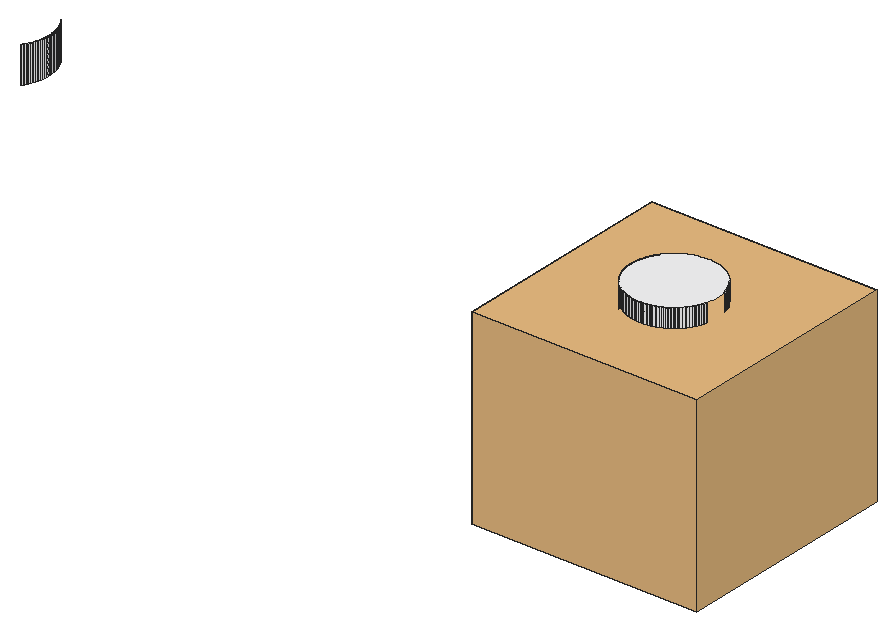
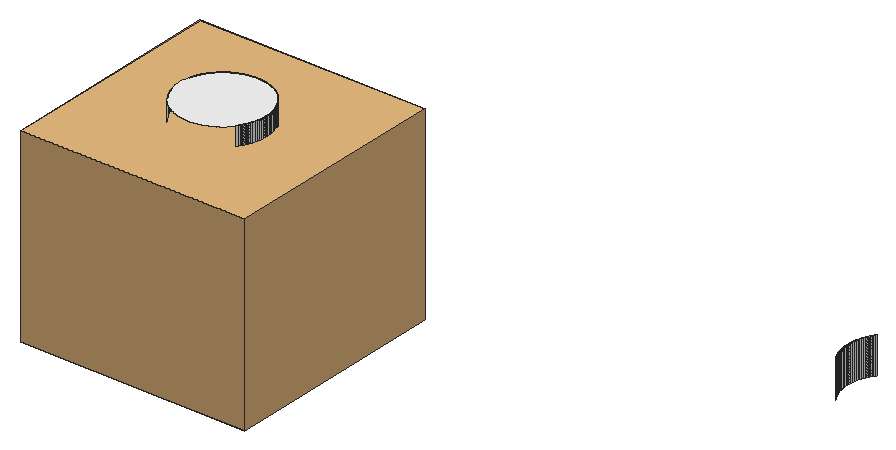
# SketchUp Ruby script. Lengths in inches.
U = 1.inch
M = Sketchup.active_model
def pt(a) = Geom::Point3d.new(a.map { |v| v * U })
def face(e, loops, mat)
  f = e.add_face(loops[0].map { |a| pt(a) })
  loops[1..].each { |l| e.add_face(l.map { |a| pt(a) }).erase! }
  f.material = f.back_material = mat if mat
  f
end
# faces: each face lists its corners as indices into pts; further lists are holes
def faces(e, pts, list, mat = nil) = list.each { |f| face(e, (f[0].is_a?(Array) ? f : [f]).map { |l| l.map { |i| pts[i] } }, mat) }
# xy, xz, yz: faces in a plane at the given z, y or x. An outline is a flat list of corners, or four numbers for a rectangle; further outlines are holes
def ring(l) = l.size == 4 ? [[l[0], l[1]], [l[2], l[1]], [l[2], l[3]], [l[0], l[3]]] : l.each_slice(2).to_a
def flat(e, list, mat, &to3) = list.each { |f| face(e, (f[0].is_a?(Array) ? f : [f]).map { |l| ring(l).map { |u, v| to3.(u, v) } }, mat) }
def xy(e, z, list, mat = nil) = flat(e, list, mat) { |x, y| [x, y, z] }
def xz(e, y, list, mat = nil) = flat(e, list, mat) { |x, z| [x, y, z] }
def yz(e, x, list, mat = nil) = flat(e, list, mat) { |y, z| [x, y, z] }
def lines(e, pts, list) = list.each { |a, b| e.add_line(pt(pts[a]), pt(pts[b])) }
# prism: a flat outline (further loops are holes) pulled along v
def prism(e, loops, v, mat = nil)
  f = face(e, loops, mat); d = Geom::Vector3d.new(v.map { |x| x * U })
  f.pushpull(f.normal.samedirection?(d) ? d.length : -d.length)
end
def box(e, o, s, mat = nil) = prism(e, [[o, [o[0] + s[0], o[1], o[2]], [o[0] + s[0], o[1] + s[1], o[2]], [o[0], o[1] + s[1], o[2]]]], [0, 0, s[2]], mat)
def at(x, y, z, deg = 0) = Geom::Transformation.translation(pt([x, y, z])) * Geom::Transformation.rotation(ORIGIN, Z_AXIS, deg.degrees)
def axes(o, x, y, z) = Geom::Transformation.new([*x, 0, *y, 0, *z, 0, *pt(o).to_a, 1])
def part(name) = M.definitions.add(name)
# library, detail: a bought-in or finely detailed component or shape, given as its bounding box
def library(name, o, s) = part(name).tap { |d| box(d.entities, o, s) }
def detail(e, o, s) = box(e.add_group.entities, o, s)
def put(e, d, t, mat = nil) = e.add_instance(d, t).tap { |i| i.material = mat if mat }
def group(e, t, mat = nil) = e.add_group.tap { |g| g.transformation = t; g.material = mat if mat }.entities
root = M.entities
M.materials.add("[Quartz Light Grey]").color = [251, 251, 252]
c1 = library("5",[-6.25,-6.25,-13.16],[15.58,15.58,13.16])
xy(root,119.5,[[161.51,250,161.35,250.02,161.28,250.03,161.12,250.05,161.04,250.07,160.97,250.08,160.89,250.1,160.81,250.125,160.74,250.15,160.67,250.17,160.59,250.2,160.45,250.26,160.375,250.29,160.3,250.33,160.24,250.36,160.03,250.48,159.97,250.53,159.9,250.57,159.6,250.82,159.55,250.88,159.49,250.93,159.4375,250.99,159.39,251.05,159.29,251.17,159.24,251.24,159.19,251.3,159.15,251.37,159.11,251.43,158.99,251.64,158.87,251.92,158.84,252,158.8125,252.07,158.79,252.15,158.77,252.22,158.75,252.3,158.73,252.375,158.72,252.45,158.7,252.53,158.69,252.61,158.68,252.6875,158.68,252.76,158.67,252.84,158.67,253.16,158.68,253.24,158.68,253.3125,158.69,253.39,158.7,253.47,158.72,253.55,158.73,253.625,158.75,253.7,158.77,253.78,158.79,253.85,158.8125,253.93,158.84,254,158.87,254.08,158.99,254.36,159.11,254.57,159.15,254.63,159.19,254.7,159.24,254.76,159.29,254.83,159.39,254.95,159.4375,255.01,159.49,255.07,159.55,255.12,159.6,255.18,159.9,255.43,159.97,255.47,160.03,255.52,160.24,255.64,160.3,255.67,160.375,255.71,160.45,255.74,160.59,255.8,160.67,255.83,160.74,255.85,160.81,255.875,160.89,255.9,160.97,255.92,161.04,255.93,161.12,255.95,161.28,255.97,161.35,255.98,161.51,256,161.82,256,162.14,255.96,162.21,255.95,162.29,255.93,162.37,255.92,162.44,255.9,162.52,255.875,162.59,255.85,162.67,255.83,162.81,255.77,162.89,255.74,162.96,255.71,163.03,255.67,163.1,255.64,163.17,255.6,163.23,255.56,163.3,255.52,163.37,255.47,163.43,255.43,163.55,255.33,163.62,255.28,163.67,255.23,163.73,255.18,163.9,255.01,164.05,254.83,164.09,254.76,164.14,254.7,164.18,254.63,164.22,254.57,164.34,254.36,164.41,254.22,164.4375,254.15,164.47,254.08,164.49,254,164.52,253.93,164.54,253.85,164.5625,253.78,164.58,253.7,164.62,253.55,164.64,253.39,164.65,253.3125,164.66,253.24,164.66,253.16,164.67,253.08,164.67,252.92,164.66,252.84,164.66,252.76,164.65,252.6875,164.64,252.61,164.62,252.45,164.58,252.3,164.5625,252.22,164.54,252.15,164.52,252.07,164.49,252,164.47,251.92,164.4375,251.85,164.41,251.78,164.34,251.64,164.22,251.43,164.18,251.37,164.14,251.3,164.09,251.24,164.05,251.17,163.9,250.99,163.73,250.82,163.67,250.77,163.62,250.72,163.55,250.67,163.43,250.57,163.37,250.53,163.3,250.48,163.23,250.44,163.17,250.4,163.1,250.36,163.03,250.33,162.96,250.29,162.89,250.26,162.81,250.23,162.67,250.17,162.59,250.15,162.52,250.125,162.44,250.1,162.37,250.08,162.29,250.07,162.21,250.05,162.14,250.04,161.82,250]],"[Quartz Light Grey]")
xz(root,250,[[161.51,117,161.59,119.5],[161.59,117,161.67,119.5],[161.67,117,161.75,119.5],[161.75,117,161.82,119.5]],"[Quartz Light Grey]")
yz(root,118.32,[[252.6875,117,252.76,119.5],[253.24,117,253.3125,119.5]],"[Quartz Light Grey]")
yz(root,118.33,[[252.84,117,252.92,119.5],[252.92,117,253,119.5],[253,117,253.08,119.5],[253.08,117,253.16,119.5]],"[Quartz Light Grey]")
yz(root,158.67,[[252.84,117,252.92,119.5],[252.92,117,253,119.5],[253,117,253.08,119.5],[253.08,117,253.16,119.5]],"[Quartz Light Grey]")
yz(root,158.68,[[252.6875,117,252.76,119.5],[253.24,117,253.3125,119.5]],"[Quartz Light Grey]")
p = [[161.2,250.04,117],[161.12,250.05,117],[161.12,250.05,119.5],[161.2,250.04,119.5],[161.28,250.03,117],[161.28,250.03,119.5],
  [161.35,250.02,117],[161.35,250.02,119.5],[161.43,250.01,117],[161.43,250.01,119.5],[161.51,250,117],[161.51,250,119.5],
  [161.9,250.01,117],[161.82,250,117],[161.82,250,119.5],[161.9,250.01,119.5],[161.98,250.02,117],[161.98,250.02,119.5],
  [162.06,250.03,117],[162.06,250.03,119.5],[162.14,250.04,117],[162.14,250.04,119.5],[162.21,250.05,117],[162.21,250.05,119.5],
  [160.74,250.15,117],[160.67,250.17,117],[160.67,250.17,119.5],[160.74,250.15,119.5],[160.81,250.125,117],[160.81,250.125,119.5],
  [160.89,250.1,117],[160.89,250.1,119.5],[160.97,250.08,117],[160.97,250.08,119.5],[161.04,250.07,117],[161.04,250.07,119.5],
  [162.29,250.07,117],[162.29,250.07,119.5],[162.37,250.08,117],[162.37,250.08,119.5],[162.44,250.1,117],[162.44,250.1,119.5],
  [162.52,250.125,117],[162.52,250.125,119.5],[162.59,250.15,117],[162.59,250.15,119.5],[162.67,250.17,117],[162.67,250.17,119.5],
  [160.52,250.23,117],[160.45,250.26,117],[160.45,250.26,119.5],[160.52,250.23,119.5],[160.59,250.2,117],[160.59,250.2,119.5],
  [162.74,250.2,117],[162.74,250.2,119.5],[162.81,250.23,117],[162.81,250.23,119.5],[162.89,250.26,117],[162.89,250.26,119.5],
  [160.3,250.33,117],[160.24,250.36,117],[160.24,250.36,119.5],[160.3,250.33,119.5],[160.375,250.29,117],[160.375,250.29,119.5],
  [162.96,250.29,117],[162.96,250.29,119.5],[163.03,250.33,117],[163.03,250.33,119.5],[163.1,250.36,117],[163.1,250.36,119.5],
  [160.1,250.44,117],[160.03,250.48,117],[160.03,250.48,119.5],[160.1,250.44,119.5],[160.17,250.4,117],[160.17,250.4,119.5],
  [163.17,250.4,117],[163.17,250.4,119.5],[163.23,250.44,117],[163.23,250.44,119.5],[163.3,250.48,117],[163.3,250.48,119.5],
  [159.97,250.53,117],[159.9,250.57,117],[159.9,250.57,119.5],[159.97,250.53,119.5],[163.37,250.53,117],[163.37,250.53,119.5],
  [163.43,250.57,117],[163.43,250.57,119.5],[159.84,250.62,117],[159.78,250.67,117],[159.78,250.67,119.5],[159.84,250.62,119.5],
  [163.49,250.62,117],[163.49,250.62,119.5],[163.55,250.67,117],[163.55,250.67,119.5],[159.72,250.72,117],[159.66,250.77,117],
  [159.66,250.77,119.5],[159.72,250.72,119.5],[163.62,250.72,117],[163.62,250.72,119.5],[163.67,250.77,117],[163.67,250.77,119.5],
  [159.6,250.82,117],[159.55,250.88,117],[159.55,250.88,119.5],[159.6,250.82,119.5],[163.73,250.82,117],[163.73,250.82,119.5],
  [163.79,250.88,117],[163.79,250.88,119.5],[159.49,250.93,117],[159.4375,250.99,117],[159.4375,250.99,119.5],[159.49,250.93,119.5],
  [163.84,250.93,117],[163.84,250.93,119.5],[163.9,250.99,117],[163.9,250.99,119.5],[159.39,251.05,117],[159.39,251.05,119.5],
  [163.95,251.05,117],[163.95,251.05,119.5],[159.34,251.11,117],[159.29,251.17,117],[159.29,251.17,119.5],[159.34,251.11,119.5],
  [164,251.11,117],[164,251.11,119.5],[164.05,251.17,117],[164.05,251.17,119.5],[117.81,251.3,117],[117.76,251.24,117],
  [117.76,251.24,119.5],[117.81,251.3,119.5],[159.24,251.24,117],[159.19,251.3,117],[159.19,251.3,119.5],[159.24,251.24,119.5],
  [164.09,251.24,117],[164.09,251.24,119.5],[164.14,251.3,117],[164.14,251.3,119.5],[117.85,251.37,117],[117.85,251.37,119.5],
  [159.15,251.37,117],[159.15,251.37,119.5],[164.18,251.37,117],[164.18,251.37,119.5],[117.89,251.43,117],[117.89,251.43,119.5],
  [117.93,251.5,117],[117.93,251.5,119.5],[159.11,251.43,117],[159.07,251.5,117],[159.07,251.5,119.5],[159.11,251.43,119.5],
  [164.22,251.43,117],[164.22,251.43,119.5],[164.26,251.5,117],[164.26,251.5,119.5],[117.97,251.57,117],[117.97,251.57,119.5],
  [159.03,251.57,117],[159.03,251.57,119.5],[164.3,251.57,117],[164.3,251.57,119.5],[118.01,251.64,117],[118.01,251.64,119.5],
  [118.04,251.71,117],[118.04,251.71,119.5],[158.99,251.64,117],[158.96,251.71,117],[158.96,251.71,119.5],[158.99,251.64,119.5],
  [164.34,251.64,117],[164.34,251.64,119.5],[164.375,251.71,117],[164.375,251.71,119.5],[118.07,251.78,117],[118.07,251.78,119.5],
  [158.93,251.78,117],[158.93,251.78,119.5],[164.41,251.78,117],[164.41,251.78,119.5],[118.1,251.85,117],[118.1,251.85,119.5],
  [158.9,251.85,117],[158.9,251.85,119.5],[164.4375,251.85,117],[164.4375,251.85,119.5],[118.13,251.92,117],[118.13,251.92,119.5],
  [118.16,252,117],[118.16,252,119.5],[158.87,251.92,117],[158.84,252,117],[158.84,252,119.5],[158.87,251.92,119.5],
  [164.47,251.92,117],[164.47,251.92,119.5],[164.49,252,117],[164.49,252,119.5],[118.1875,252.07,117],[118.1875,252.07,119.5],
  [158.8125,252.07,117],[158.8125,252.07,119.5],[164.52,252.07,117],[164.52,252.07,119.5],[118.21,252.15,117],[118.21,252.15,119.5],
  [118.23,252.22,117],[118.23,252.22,119.5],[158.79,252.15,117],[158.77,252.22,117],[158.77,252.22,119.5],[158.79,252.15,119.5],
  [164.54,252.15,117],[164.54,252.15,119.5],[164.5625,252.22,117],[164.5625,252.22,119.5],[118.25,252.3,117],[118.25,252.3,119.5],
  [158.75,252.3,117],[158.75,252.3,119.5],[118.27,252.375,117],[118.27,252.375,119.5],[158.73,252.375,117],[158.73,252.375,119.5],
  [118.28,252.45,117],[118.28,252.45,119.5],[158.72,252.45,117],[158.72,252.45,119.5],[118.3,252.53,117],[118.3,252.53,119.5],
  [118.31,252.61,117],[118.31,252.61,119.5],[158.7,252.53,117],[158.69,252.61,117],[158.69,252.61,119.5],[158.7,252.53,119.5],
  [118.32,252.6875,117],[118.32,252.6875,119.5],[158.68,252.6875,117],[158.68,252.6875,119.5],[118.33,252.84,117],[118.32,252.76,117],
  [118.32,252.76,119.5],[118.33,252.84,119.5],[158.68,252.76,117],[158.67,252.84,117],[158.67,252.84,119.5],[158.68,252.76,119.5],
  [118.32,253.24,117],[118.33,253.16,117],[118.33,253.16,119.5],[118.32,253.24,119.5],[158.67,253.16,117],[158.68,253.24,117],
  [158.68,253.24,119.5],[158.67,253.16,119.5],[118.31,253.39,117],[118.32,253.3125,117],[118.32,253.3125,119.5],[118.31,253.39,119.5],
  [158.68,253.3125,117],[158.69,253.39,117],[158.69,253.39,119.5],[158.68,253.3125,119.5],[118.3,253.47,117],[118.3,253.47,119.5],
  [158.7,253.47,117],[158.7,253.47,119.5],[118.27,253.625,117],[118.28,253.55,117],[118.28,253.55,119.5],[118.27,253.625,119.5],
  [158.72,253.55,117],[158.72,253.55,119.5],[158.73,253.625,117],[158.73,253.625,119.5],[118.25,253.7,117],[118.25,253.7,119.5],
  [158.75,253.7,117],[158.75,253.7,119.5],[118.23,253.78,117],[118.23,253.78,119.5],[158.77,253.78,117],[158.77,253.78,119.5],
  [118.21,253.85,117],[118.21,253.85,119.5],[158.79,253.85,117],[158.79,253.85,119.5],[118.16,254,117],[118.1875,253.93,117],
  [118.1875,253.93,119.5],[118.16,254,119.5],[158.8125,253.93,117],[158.8125,253.93,119.5],[158.84,254,117],[158.84,254,119.5],
  [164.49,254,117],[164.52,253.93,117],[164.52,253.93,119.5],[164.49,254,119.5],[164.54,253.85,117],[164.54,253.85,119.5],
  [118.13,254.08,117],[118.13,254.08,119.5],[158.87,254.08,117],[158.87,254.08,119.5],[164.47,254.08,117],[164.47,254.08,119.5],
  [118.07,254.22,117],[118.1,254.15,117],[118.1,254.15,119.5],[118.07,254.22,119.5],[158.9,254.15,117],[158.9,254.15,119.5],
  [158.93,254.22,117],[158.93,254.22,119.5],[164.41,254.22,117],[164.4375,254.15,117],[164.4375,254.15,119.5],[164.41,254.22,119.5],
  [118.04,254.29,117],[118.04,254.29,119.5],[158.96,254.29,117],[158.96,254.29,119.5],[164.375,254.29,117],[164.375,254.29,119.5],
  [118.01,254.36,117],[118.01,254.36,119.5],[158.99,254.36,117],[158.99,254.36,119.5],[164.34,254.36,117],[164.34,254.36,119.5],
  [117.93,254.5,117],[117.97,254.43,117],[117.97,254.43,119.5],[117.93,254.5,119.5],[159.03,254.43,117],[159.03,254.43,119.5],
  [159.07,254.5,117],[159.07,254.5,119.5],[164.26,254.5,117],[164.3,254.43,117],[164.3,254.43,119.5],[164.26,254.5,119.5],
  [117.89,254.57,117],[117.89,254.57,119.5],[159.11,254.57,117],[159.11,254.57,119.5],[164.22,254.57,117],[164.22,254.57,119.5],
  [117.81,254.7,117],[117.85,254.63,117],[117.85,254.63,119.5],[117.81,254.7,119.5],[159.15,254.63,117],[159.15,254.63,119.5],
  [159.19,254.7,117],[159.19,254.7,119.5],[164.14,254.7,117],[164.18,254.63,117],[164.18,254.63,119.5],[164.14,254.7,119.5],
  [117.76,254.76,117],[117.76,254.76,119.5],[159.24,254.76,117],[159.24,254.76,119.5],[164.09,254.76,117],[164.09,254.76,119.5],
  [159.29,254.83,117],[159.29,254.83,119.5],[164.05,254.83,117],[164.05,254.83,119.5]]
faces(root,p,[[0,1,2,3],[4,0,3,5],[6,4,5,7],[8,6,7,9],[10,8,9,11],[12,13,14,15],[16,12,15,17],[18,16,17,19],
  [20,18,19,21],[22,20,21,23],[24,25,26,27],[28,24,27,29],[30,28,29,31],[32,30,31,33],[34,32,33,35],[1,34,35,2],
  [36,22,23,37],[38,36,37,39],[40,38,39,41],[42,40,41,43],[44,42,43,45],[46,44,45,47],[48,49,50,51],[52,48,51,53],
  [25,52,53,26],[54,46,47,55],[56,54,55,57],[58,56,57,59],[60,61,62,63],[64,60,63,65],[49,64,65,50],[66,58,59,67],
  [68,66,67,69],[70,68,69,71],[72,73,74,75],[76,72,75,77],[61,76,77,62],[78,70,71,79],[80,78,79,81],[82,80,81,83],
  [84,85,86,87],[73,84,87,74],[88,82,83,89],[90,88,89,91],[92,93,94,95],[85,92,95,86],[96,90,91,97],[98,96,97,99],
  [100,101,102,103],[93,100,103,94],[104,98,99,105],[106,104,105,107],[108,109,110,111],[101,108,111,102],[112,106,107,113],[114,112,113,115],
  [116,117,118,119],[109,116,119,110],[120,114,115,121],[122,120,121,123],[117,124,125,118],[126,122,123,127],[128,129,130,131],[124,128,131,125],
  [132,126,127,133],[134,132,133,135],[136,137,138,139],[140,141,142,143],[129,140,143,130],[144,134,135,145],[146,144,145,147],[148,136,139,149],
  [141,150,151,142],[152,146,147,153],[154,148,149,155],[156,154,155,157],[158,159,160,161],[150,158,161,151],[162,152,153,163],[164,162,163,165],
  [166,156,157,167],[159,168,169,160],[170,164,165,171],[172,166,167,173],[174,172,173,175],[176,177,178,179],[168,176,179,169],[180,170,171,181],
  [182,180,181,183],[184,174,175,185],[177,186,187,178],[188,182,183,189],[190,184,185,191],[186,192,193,187],[194,188,189,195],[196,190,191,197],
  [198,196,197,199],[200,201,202,203],[192,200,203,193],[204,194,195,205],[206,204,205,207],[208,198,199,209],[201,210,211,202],[212,206,207,213],
  [214,208,209,215],[216,214,215,217],[218,219,220,221],[210,218,221,211],[222,212,213,223],[224,222,223,225],[226,216,217,227],[219,228,229,220],
  [230,226,227,231],[228,232,233,229],[234,230,231,235],[232,236,237,233],[238,234,235,239],[240,238,239,241],[242,243,244,245],[236,242,245,237],
  [246,240,241,247],[243,248,249,244],[250,251,252,253],[254,255,256,257],[258,259,260,261],[262,263,264,265],[266,267,268,269],[270,271,272,273],
  [274,266,269,275],[271,276,277,272],[278,279,280,281],[279,274,275,280],[276,282,283,277],[282,284,285,283],[286,278,281,287],[284,288,289,285],
  [290,286,287,291],[288,292,293,289],[294,290,291,295],[292,296,297,293],[298,299,300,301],[299,294,295,300],[296,302,303,297],[302,304,305,303],
  [306,307,308,309],[307,310,311,308],[312,298,301,313],[304,314,315,305],[316,306,309,317],[318,319,320,321],[319,312,313,320],[314,322,323,315],
  [322,324,325,323],[326,327,328,329],[327,316,317,328],[330,318,321,331],[324,332,333,325],[334,326,329,335],[336,330,331,337],[332,338,339,333],
  [340,334,335,341],[342,343,344,345],[343,336,337,344],[338,346,347,339],[346,348,349,347],[350,351,352,353],[351,340,341,352],[354,342,345,355],
  [348,356,357,349],[358,350,353,359],[360,361,362,363],[361,354,355,362],[356,364,365,357],[364,366,367,365],[368,369,370,371],[369,358,359,370],
  [372,360,363,373],[366,374,375,367],[376,368,371,377],[374,378,379,375],[380,376,377,381]],"[Quartz Light Grey]")
put(root,c1,at(160.13,251.46,118.25),"[Quartz Light Grey]")
